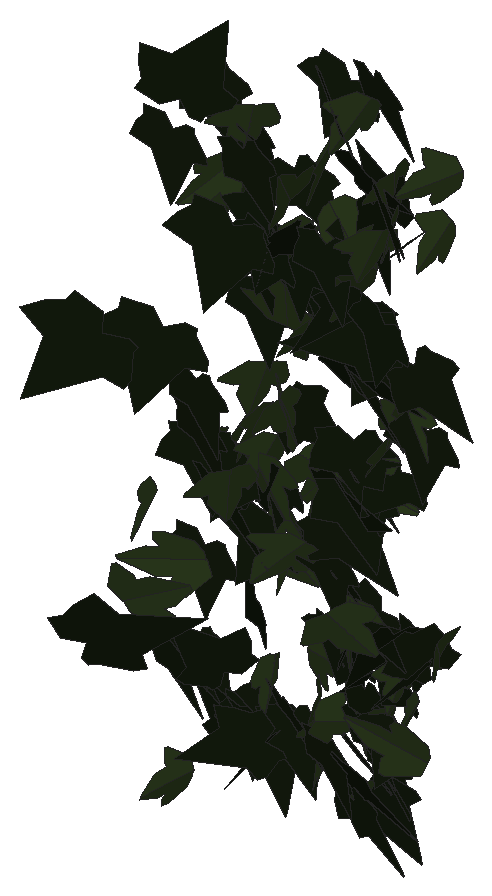
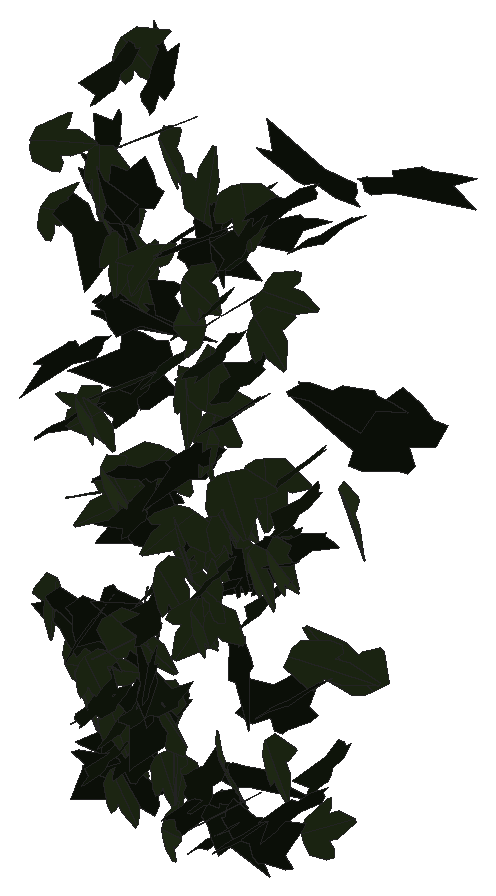
# SketchUp Ruby script. Lengths in inches.
U = 1.inch
M = Sketchup.active_model
def pt(a) = Geom::Point3d.new(a.map { |v| v * U })
def face(e, loops, mat)
  f = e.add_face(loops[0].map { |a| pt(a) })
  loops[1..].each { |l| e.add_face(l.map { |a| pt(a) }).erase! }
  f.material = f.back_material = mat if mat
  f
end
# faces: each face lists its corners as indices into pts; further lists are holes
def faces(e, pts, list, mat = nil) = list.each { |f| face(e, (f[0].is_a?(Array) ? f : [f]).map { |l| l.map { |i| pts[i] } }, mat) }
# xy, xz, yz: faces in a plane at the given z, y or x. An outline is a flat list of corners, or four numbers for a rectangle; further outlines are holes
def ring(l) = l.size == 4 ? [[l[0], l[1]], [l[2], l[1]], [l[2], l[3]], [l[0], l[3]]] : l.each_slice(2).to_a
def flat(e, list, mat, &to3) = list.each { |f| face(e, (f[0].is_a?(Array) ? f : [f]).map { |l| ring(l).map { |u, v| to3.(u, v) } }, mat) }
def xy(e, z, list, mat = nil) = flat(e, list, mat) { |x, y| [x, y, z] }
def xz(e, y, list, mat = nil) = flat(e, list, mat) { |x, z| [x, y, z] }
def yz(e, x, list, mat = nil) = flat(e, list, mat) { |y, z| [x, y, z] }
def lines(e, pts, list) = list.each { |a, b| e.add_line(pt(pts[a]), pt(pts[b])) }
# prism: a flat outline (further loops are holes) pulled along v
def prism(e, loops, v, mat = nil)
  f = face(e, loops, mat); d = Geom::Vector3d.new(v.map { |x| x * U })
  f.pushpull(f.normal.samedirection?(d) ? d.length : -d.length)
end
def box(e, o, s, mat = nil) = prism(e, [[o, [o[0] + s[0], o[1], o[2]], [o[0] + s[0], o[1] + s[1], o[2]], [o[0], o[1] + s[1], o[2]]]], [0, 0, s[2]], mat)
def at(x, y, z, deg = 0) = Geom::Transformation.translation(pt([x, y, z])) * Geom::Transformation.rotation(ORIGIN, Z_AXIS, deg.degrees)
def axes(o, x, y, z) = Geom::Transformation.new([*x, 0, *y, 0, *z, 0, *pt(o).to_a, 1])
def part(name) = M.definitions.add(name)
# library, detail: a bought-in or finely detailed component or shape, given as its bounding box
def library(name, o, s) = part(name).tap { |d| box(d.entities, o, s) }
def detail(e, o, s) = box(e.add_group.entities, o, s)
def put(e, d, t, mat = nil) = e.add_instance(d, t).tap { |i| i.material = mat if mat }
def group(e, t, mat = nil) = e.add_group.tap { |g| g.transformation = t; g.material = mat if mat }.entities
root = M.entities
M.materials.add("1026 AP 7946 SUNNY SIDE UP").color = [254, 231, 186]
M.materials.add("efeu1").color = [18, 25, 13]
M.materials.add("efeu2").color = [43, 57, 29]
c1 = part("ivyleaf_9")
p = [[1.54,2.16,1.25],[1.36,2.04,1.19],[-0.21,0.99,0.68],[-0.71,1.11,0.82],[-0.85,0.86,0.67],[-0.8,0.17,0.21],
  [-0.9,-0.01,0.1],[-0.67,-0.16,-0.02],[-0.08,-0.08,-0.05],[-0.03,-0.6,-0.4],[0.65,-0.88,-0.66],[0.83,-0.6,-0.49],
  [1.29,-0.42,-0.43],[1.8125,-0.07,-0.26],[1.21,0.44,0.15]]
faces(c1.entities,p,[[0,1,2,3,4,5,6,7,8,9,10,11,12,13,14]],"efeu1")
c2 = part("ivyleaf_10")
p = [[0,0.5,-0.03],[-0.0625,2.02,-0.43],[-0.19,2.01,-0.46],[-0.54,1.05,-0.29],[-0.52,0.625,-0.18],[-0.83,0.76,-0.28],
  [-1.16,0.64,-0.33],[-1.15,0.33,-0.24],[-0.77,-0.39,0.02],[-0.3,-0.51,0.16],[0.04,-0.48,0.23],[-0.02,2.01,-0.4375],
  [-0.06,2.01,-0.43],[0.04,-0.49,0.23],[0.67,-0.49,0.14],[1.38,0.36,-0.2],[1.375,0.51,-0.24],[0.81,0.65,-0.19],
  [0.62,0.59,-0.15],[0.6,1.09,-0.28],[0.5,1.23,-0.31]]
faces(c2.entities,p,[[0,1,2,3,4,5,6,7,8,9,10],[11,12,0,13,14,15,16,17,18,19,20]],"efeu2")
put(root,c1,axes([119.27,207.23,283.47],[0.0723,0.01785,0.46303],[0.70235,0.05061,-0.04886],[-0.08206,0.44886,-0.01025]),"1026 AP 7946 SUNNY SIDE UP")
put(root,c1,axes([118.96,207.77,288.06],[-0.55273,-0.26197,0.11681],[-0.11258,-0.09563,-0.45093],[0.43547,-0.35723,0.03168]),"1026 AP 7946 SUNNY SIDE UP")
put(root,c2,axes([121.6,209.79,283.51],[-0.33142,-0.22889,-0.23164],[0.26923,0.14544,-0.31887],[0.42498,-0.27064,0.02137]),"1026 AP 7946 SUNNY SIDE UP")
put(root,c2,axes([118.09,209.97,284.15],[0.24212,-0.34202,-0.03713],[-0.02534,0.03014,-0.38622],[0.53986,0.15481,-0.00147]),"1026 AP 7946 SUNNY SIDE UP")
put(root,c1,axes([119.03,210.66,288.52],[-0.31904,-0.36893,0.03508],[0.00177,-0.04182,-0.43345],[0.58288,-0.2018,0.02052]),"1026 AP 7946 SUNNY SIDE UP")
put(root,c2,axes([117.99,210.81,279.3],[0.00507,-0.02154,0.37214],[0.06882,-0.3587,-0.02453],[0.56503,0.04388,-0.00035]),"1026 AP 7946 SUNNY SIDE UP")
put(root,c1,axes([117.71,210.74,286.4],[-0.47629,-0.266,-0.09673],[0.14411,0.03517,-0.41368],[0.41865,-0.31472,0.03235]),"1026 AP 7946 SUNNY SIDE UP")
put(root,c2,axes([119.04,210.58,284.55],[-0.23896,-0.35345,-0.04487],[0.04278,0.03351,-0.39598],[0.55796,-0.15395,0.01114]),"1026 AP 7946 SUNNY SIDE UP")
put(root,c2,axes([117.3125,210.67,281.95],[-0.39183,-0.04375,0.2858],[0.41038,0.10184,0.25841],[-0.1642,0.35893,-0.03618]),"1026 AP 7946 SUNNY SIDE UP")
put(root,c1,axes([121.41,211.1,287.61],[-0.03806,-0.30393,0.19273],[-0.02274,-0.18825,-0.3152],[0.56214,-0.02819,0.0003]),"1026 AP 7946 SUNNY SIDE UP")
put(root,c1,axes([118.55,211.06,281.09],[0.1272,0.0928,0.35483],[-0.48936,-0.15313,0.1171],[0.27245,-0.31838,0.04466]),"1026 AP 7946 SUNNY SIDE UP")
put(root,c1,axes([119.24,211.25,288.06],[-0.10866,-0.26363,0.23482],[0.00898,-0.2347,-0.27742],[0.54946,-0.0483,0.05097]),"1026 AP 7946 SUNNY SIDE UP")
put(root,c2,axes([120.97,211.16,290.9375],[-0.11826,-0.28478,0.22358],[0.00122,-0.22352,-0.30095],[0.56454,-0.05917,0.04749]),"1026 AP 7946 SUNNY SIDE UP")
put(root,c2,axes([119.76,211.16,283.41],[-0.25485,-0.22405,0.22789],[-0.17352,-0.19411,-0.28534],[0.46518,-0.19516,0.01841]),"1026 AP 7946 SUNNY SIDE UP")
put(root,c1,axes([120.3,211.18,280.42],[0.15225,-0.31296,0.08945],[0.0206,-0.08862,-0.33773],[0.51102,0.09681,-0.01304]),"1026 AP 7946 SUNNY SIDE UP")
put(root,c2,axes([119.6,211.31,288.96],[-0.05659,-0.29494,-0.28113],[-0.03716,-0.27027,0.30443],[-0.62894,0.0425,0.00731]),"1026 AP 7946 SUNNY SIDE UP")
put(root,c1,axes([120.33,211.37,290.57],[-0.01449,-0.11425,0.40246],[0.04558,-0.39061,-0.11907],[0.63937,0.02526,0.01761]),"1026 AP 7946 SUNNY SIDE UP")
put(root,c1,axes([119.11,211.24,280.04],[-0.46237,-0.05005,0.15696],[-0.2235,-0.0673,-0.3052],[0.1177,-0.3244,0.03708]),"1026 AP 7946 SUNNY SIDE UP")
put(root,c1,axes([117.46,211.3125,289.26],[-0.08111,-0.34399,0.06496],[-0.00048,-0.06566,-0.3586],[0.55047,-0.05075,0.00926]),"1026 AP 7946 SUNNY SIDE UP")
put(root,c1,axes([119.65,211.32,288.41],[-0.21655,0.11551,-0.31747],[0.17231,-0.29962,-0.16755],[-0.48898,-0.15674,0.08155]),"1026 AP 7946 SUNNY SIDE UP")
put(root,c1,axes([119.34,211.37,288.67],[-0.21556,0.05674,-0.38318],[0.46434,-0.22964,-0.14943],[-0.36743,-0.32349,0.03596]),"1026 AP 7946 SUNNY SIDE UP")
put(root,c1,axes([117.88,211.32,285.35],[0.08751,-0.33903,0.04372],[0.00471,-0.04446,-0.35417],[0.53761,0.05558,-0.00402]),"1026 AP 7946 SUNNY SIDE UP")
put(root,c1,axes([121.17,211.41,289.31],[0.22112,-0.10123,-0.35227],[0.47956,-0.15517,0.17593],[-0.28894,-0.33501,0.0224]),"1026 AP 7946 SUNNY SIDE UP")
put(root,c1,axes([120.86,211.2,279.66],[0.32279,-0.2569,-0.08403],[-0.07729,0.06327,-0.3384],[0.41601,0.21108,0.00233]),"1026 AP 7946 SUNNY SIDE UP")
put(root,c2,axes([121.82,211.1875,280.81],[-0.14903,-0.01053,-0.36355],[-0.54968,0.05348,0.09541],[0.077,0.36141,-0.02255]),"1026 AP 7946 SUNNY SIDE UP")
put(root,c1,axes([117.84,211.4,284.7],[0.14055,-0.31672,0.10267],[0.03789,-0.09861,-0.33958],[0.52156,0.09251,-0.003]),"1026 AP 7946 SUNNY SIDE UP")
put(root,c1,axes([118.19,211.35,283.84],[0.34368,-0.33159,0.07424],[0.03544,-0.07358,-0.40898],[0.53303,0.21869,-0.02068]),"1026 AP 7946 SUNNY SIDE UP")
put(root,c1,axes([120.58,211.3,280.02],[0.42716,-0.18369,0.14825],[0.16073,-0.10662,-0.33719],[0.33095,0.28886,-0.02758]),"1026 AP 7946 SUNNY SIDE UP")
put(root,c1,axes([118.7,211.38,289.3125],[0.16333,-0.34209,-0.02416],[-0.02073,0.01847,-0.36813],[0.53857,0.10446,-0.00684]),"1026 AP 7946 SUNNY SIDE UP")
put(root,c2,axes([117.68,211.38,282.41],[0.16931,-0.00521,-0.35469],[-0.52703,-0.08413,-0.10717],[-0.12389,0.35077,-0.02881]),"1026 AP 7946 SUNNY SIDE UP")
put(root,c1,axes([120.11,211.46,288.24],[0.02721,-0.35324,0.01497],[0.00014,-0.01655,-0.36444],[0.55605,0.01729,-0.00064]),"1026 AP 7946 SUNNY SIDE UP")
put(root,c1,axes([117.23,211.42,280.86],[0.23734,-0.29354,0.04164],[0.00824,-0.04458,-0.33992],[0.4662,0.15023,-0.01519]),"1026 AP 7946 SUNNY SIDE UP")
put(root,c2,axes([121.04,211.4,288.74],[-0.1834,-0.32732,0.08032],[-0.01571,-0.08108,-0.358],[0.52954,-0.11577,0.0172]),"1026 AP 7946 SUNNY SIDE UP")
put(root,c2,axes([120.1,211.46,289.75],[0.20736,-0.31965,0.13025],[0.06892,-0.12064,-0.35689],[0.53717,0.13887,-0.00449]),"1026 AP 7946 SUNNY SIDE UP")
put(root,c1,axes([117.71,211.2,289.98],[-0.46698,0.1942,0.22772],[0.32132,-0.08767,0.36349],[0.33106,0.35902,-0.03158]),"1026 AP 7946 SUNNY SIDE UP")
put(root,c1,axes([119,211.64,283.17],[-0.28684,-0.25382,0.13022],[-0.02858,-0.14118,-0.31631],[0.44595,-0.1723,0.06348]),"1026 AP 7946 SUNNY SIDE UP")
put(root,c2,axes([119.375,211.32,285.52],[-0.09944,-0.30369,-0.15758],[0.10038,0.14044,-0.31721],[0.52394,-0.08455,0.03087]),"1026 AP 7946 SUNNY SIDE UP")
put(root,c2,axes([120.27,211.2,280.82],[-0.05776,-0.09502,-0.33484],[0.26367,0.2783,-0.10189],[0.46166,-0.17084,0.0163]),"1026 AP 7946 SUNNY SIDE UP")
put(root,c1,axes([117.875,211.54,284.32],[-0.1917,-0.3008,-0.1039],[0.07119,0.0886,-0.33374],[0.49289,-0.12979,0.00779]),"1026 AP 7946 SUNNY SIDE UP")
put(root,c1,axes([120.96,211.61,286.93],[-0.45254,0.00304,0.23472],[-0.35611,-0.04402,-0.29438],[0.03924,-0.36441,0.03535]),"1026 AP 7946 SUNNY SIDE UP")
put(root,c1,axes([120.52,211.68,287.36],[0.021,0.08055,-0.36137],[-0.02984,-0.35083,-0.08568],[-0.56584,0.02149,-0.00889]),"1026 AP 7946 SUNNY SIDE UP")
put(root,c2,axes([120.29,211.72,282.1875],[0.13277,-0.1327,0.33736],[0.34978,-0.24263,-0.16142],[0.43308,0.23664,0.02694]),"1026 AP 7946 SUNNY SIDE UP")
put(root,c2,axes([120.41,211.73,287.49],[-0.11359,-0.24495,-0.26929],[-0.0791,-0.25565,0.26102],[-0.55608,0.0864,0.01788]),"1026 AP 7946 SUNNY SIDE UP")
put(root,c1,axes([120.58,211.61,280.76],[0.24396,-0.27932,-0.01255],[-0.03559,-0.00048,-0.32852],[0.43808,0.15551,-0.0197]),"1026 AP 7946 SUNNY SIDE UP")
put(root,c1,axes([121.1,211.79,280.6],[-0.1552,-0.27336,0.16236],[-0.0242,-0.16238,-0.2981],[0.49679,-0.09331,0.0362]),"1026 AP 7946 SUNNY SIDE UP")
put(root,c2,axes([119.55,211.32,285.18],[-0.15586,0.16681,-0.32485],[-0.2027,0.28947,0.20059],[0.52444,0.16146,-0.01902]),"1026 AP 7946 SUNNY SIDE UP")
put(root,c1,axes([119.86,211.77,283.11],[0.06685,-0.35386,0.0836],[-0.00272,-0.08392,-0.36747],[0.57156,0.04099,-0.01153]),"1026 AP 7946 SUNNY SIDE UP")
put(root,c1,axes([120.2,211.59,283.77],[-0.05483,-0.19776,-0.28665],[0.32329,0.20981,-0.17967],[0.42668,-0.18438,0.0993]),"1026 AP 7946 SUNNY SIDE UP")
put(root,c1,axes([118.85,211.43,282.16],[0.17233,-0.02558,-0.34789],[-0.50876,0.0964,-0.11519],[0.15649,0.34156,0.00863]),"1026 AP 7946 SUNNY SIDE UP")
put(root,c1,axes([121.09,211.7,282.22],[-0.0476,0.24807,-0.26669],[0.05207,-0.25817,-0.25896],[-0.56297,-0.04485,-0.00141]),"1026 AP 7946 SUNNY SIDE UP")
put(root,c2,axes([118.04,211.7,280.93],[0.07461,-0.34398,0.01441],[-0.00343,-0.01639,-0.35779],[0.54145,0.0473,-0.00425]),"1026 AP 7946 SUNNY SIDE UP")
put(root,c1,axes([120.34,211.77,284.22],[-0.08114,-0.32891,-0.12629],[0.06613,0.11533,-0.34155],[0.54694,-0.06274,0.02256]),"1026 AP 7946 SUNNY SIDE UP")
put(root,c1,axes([118.6,211.97,287.92],[-0.18784,-0.24877,0.22669],[-0.07059,-0.2211,-0.2821],[0.51892,-0.12013,0.04368]),"1026 AP 7946 SUNNY SIDE UP")
put(root,c1,axes([120.71,211.7,279.68],[-0.17972,-0.11894,-0.3288],[0.41389,0.1817,-0.16615],[0.33833,-0.28546,0.0286]),"1026 AP 7946 SUNNY SIDE UP")
put(root,c1,axes([121.62,211.77,281.92],[-0.31121,0.18615,-0.17988],[0.12604,-0.16581,-0.27502],[-0.38221,-0.20625,0.05577]),"1026 AP 7946 SUNNY SIDE UP")
put(root,c1,axes([120.55,211.84,279.875],[0.34606,-0.25477,0.02838],[0.00079,0.03864,0.34606],[-0.40318,-0.2186,0.02504]),"1026 AP 7946 SUNNY SIDE UP")
put(root,c1,axes([119.93,211.86,283.92],[0.12855,-0.08863,0.35421],[0.29583,-0.28901,-0.12435],[0.47439,0.20425,-0.01844]),"1026 AP 7946 SUNNY SIDE UP")
put(root,c1,axes([119.14,211.93,287.6],[0.01507,-0.32432,0.14133],[0.02085,-0.13865,-0.33495],[0.55444,0.01403,0.00875]),"1026 AP 7946 SUNNY SIDE UP")
put(root,c2,axes([119.29,211.91,288.04],[0.02238,-0.26559,0.24009],[0.06124,-0.23216,-0.2746],[0.55379,0.03641,0.02066]),"1026 AP 7946 SUNNY SIDE UP")
put(root,c2,axes([118.72,211.73,284.14],[-0.4702,0.12526,-0.14769],[0.18001,-0.09661,-0.33188],[-0.24023,-0.31756,0.04039]),"1026 AP 7946 SUNNY SIDE UP")
put(root,c1,axes([120.09,211.72,286.3125],[0.47502,-0.08576,0.18557],[0.25315,-0.08971,-0.32183],[0.18642,0.34035,-0.03581]),"1026 AP 7946 SUNNY SIDE UP")
put(root,c1,axes([120.66,211.87,290.9375],[0.2439,-0.3204,0.07242],[0.0184,-0.07432,-0.36649],[0.51607,0.15408,-0.02116]),"1026 AP 7946 SUNNY SIDE UP")
put(root,c2,axes([117.82,211.89,284.19],[0.14594,-0.27935,0.17523],[0.06611,-0.16681,-0.30401],[0.51131,0.1013,-0.01071]),"1026 AP 7946 SUNNY SIDE UP")
put(root,c2,axes([118.76,211.87,284.43],[-0.10013,-0.29984,0.15174],[0.01551,-0.15328,-0.31433],[0.52624,-0.05253,0.03813]),"1026 AP 7946 SUNNY SIDE UP")
put(root,c2,axes([120.7,211.81,279.6],[-0.02735,-0.32044,0.0741],[-0.00533,-0.07367,-0.33103],[0.517,-0.01771,0.00051]),"1026 AP 7946 SUNNY SIDE UP")
put(root,c1,axes([118.86,211.81,279.77],[-0.24732,0.23176,-0.21318],[0.15019,-0.18618,-0.28887],[-0.46633,-0.18288,0.02002]),"1026 AP 7946 SUNNY SIDE UP")
put(root,c1,axes([118.25,212,283.82],[-0.25079,-0.26653,0.12546],[-0.06848,-0.11729,-0.31992],[0.45666,-0.16397,0.02093]),"1026 AP 7946 SUNNY SIDE UP")
put(root,c2,axes([118.58,211.92,284.84],[0.10921,-0.32184,0.1678],[0.03749,-0.16327,-0.33999],[0.56725,0.07275,-0.00983]),"1026 AP 7946 SUNNY SIDE UP")
put(root,c2,axes([118.47,211.8,289.6875],[-0.29225,-0.30524,0.02096],[0.00556,-0.02797,-0.36789],[0.48118,-0.18507,0.01698]),"1026 AP 7946 SUNNY SIDE UP")
put(root,c2,axes([117.85,211.96,288.47],[0.13835,0.18126,-0.2982],[-0.27667,-0.23336,-0.20628],[-0.46187,0.19408,0.03424]),"1026 AP 7946 SUNNY SIDE UP")
put(root,c1,axes([117.9,211.96,283.52],[0.12413,-0.32061,0.07462],[0.01418,-0.07422,-0.34047],[0.51728,0.07897,-0.00857]),"1026 AP 7946 SUNNY SIDE UP")
put(root,c1,axes([121.58,211.86,281.89],[-0.0151,0.03674,0.33041],[-0.50678,0.01333,-0.01144],[-0.02281,-0.32039,0.03551]),"1026 AP 7946 SUNNY SIDE UP")
put(root,c2,axes([120.94,211.98,288.93],[0.2507,-0.26976,0.19407],[0.14754,-0.16513,-0.32376],[0.49731,0.18498,-0.00177]),"1026 AP 7946 SUNNY SIDE UP")
put(root,c1,axes([117.71,211.86,289.96],[0.04426,-0.33652,-0.1402],[-0.0208,0.13354,-0.34711],[0.56928,0.03104,-0.00178]),"1026 AP 7946 SUNNY SIDE UP")
put(root,c2,axes([120.75,211.88,280.76],[-0.04993,-0.3275,0.04475],[0.00175,-0.04561,-0.33919],[0.51986,-0.0313,0.00544]),"1026 AP 7946 SUNNY SIDE UP")
put(root,c1,axes([118.73,211.97,279.54],[0.00266,-0.32496,0.0031],[0.00319,-0.00485,-0.3348],[0.51102,0.00172,0.00208]),"1026 AP 7946 SUNNY SIDE UP")
put(root,c1,axes([118.4,212,283.7],[-0.00986,0.07829,0.34962],[0.08456,-0.33469,0.07871],[0.54039,0.0538,-0.00594]),"1026 AP 7946 SUNNY SIDE UP")
put(root,c2,axes([119.07,212.04,282.85],[0.10587,-0.27765,0.21302],[0.12699,-0.19388,-0.29419],[0.53085,0.10175,0.02789]),"1026 AP 7946 SUNNY SIDE UP")
put(root,c1,axes([118.91,212.01,280.25],[0.23623,-0.26016,0.14387],[0.07262,-0.13573,-0.3092],[0.45969,0.15514,-0.02509]),"1026 AP 7946 SUNNY SIDE UP")
put(root,c2,axes([120.56,211.9,282.15],[-0.31543,-0.02273,0.29731],[-0.42343,-0.11464,-0.20271],[0.16763,-0.33236,0.04741]),"1026 AP 7946 SUNNY SIDE UP")
put(root,c1,axes([120.51,212.02,288.74],[-0.18522,-0.01736,-0.37564],[0.56556,-0.07036,-0.11669],[-0.09713,-0.37657,0.03684]),"1026 AP 7946 SUNNY SIDE UP")
put(root,c2,axes([118.61,212.05,280.71],[0.32978,-0.20176,0.23159],[0.22347,-0.17716,-0.2999],[0.42063,0.2523,-0.02224]),"1026 AP 7946 SUNNY SIDE UP")
put(root,c1,axes([120.26,211.99,285.96],[0.29068,-0.27561,0.09882],[0.05006,-0.09568,-0.34141],[0.45695,0.18581,-0.02546]),"1026 AP 7946 SUNNY SIDE UP")
put(root,c2,axes([121.27,211.91,281.02],[0.17149,-0.30029,-0.01772],[-0.02628,0.0104,-0.32883],[0.47207,0.10967,-0.01187]),"1026 AP 7946 SUNNY SIDE UP")
put(root,c1,axes([117.41,212.1,282.2],[-0.06396,-0.33941,0.07238],[0.00933,-0.07335,-0.35228],[0.54555,-0.03854,0.01451]),"1026 AP 7946 SUNNY SIDE UP")
put(root,c1,axes([121.2,212.15,281.72],[-0.13026,-0.0184,0.33457],[-0.19343,-0.30858,-0.05212],[0.47367,-0.13107,0.07073]),"1026 AP 7946 SUNNY SIDE UP")
put(root,c1,axes([120.16,212.01,284.87],[-0.09902,-0.33279,-0.13222],[0.06808,0.1203,-0.34768],[0.55563,-0.07405,0.01904]),"1026 AP 7946 SUNNY SIDE UP")
put(root,c1,axes([119.3,211.76,285.29],[0.14838,-0.15241,-0.32027],[-0.15223,0.29683,-0.17895],[0.52142,0.13003,0.03889]),"1026 AP 7946 SUNNY SIDE UP")
put(root,c1,axes([120.67,212.08,280.05],[0.13697,-0.29361,0.07294],[0.017,-0.07234,-0.31577],[0.47523,0.08722,-0.00972]),"1026 AP 7946 SUNNY SIDE UP")
put(root,c1,axes([120.15,212.09,289.13],[0.14021,-0.15597,0.31466],[0.28939,-0.24562,-0.18546],[0.45651,0.2036,0.02093]),"1026 AP 7946 SUNNY SIDE UP")
put(root,c2,axes([119.71,211.99,280.27],[-0.04954,-0.32992,0.03169],[-0.0002,-0.03277,-0.34161],[0.5213,-0.03137,0.00288]),"1026 AP 7946 SUNNY SIDE UP")
put(root,c2,axes([118.72,212.09,283.34],[0.05302,-0.04502,0.35465],[0.49038,-0.14864,-0.05233],[0.2408,0.31262,0.02848]),"1026 AP 7946 SUNNY SIDE UP")
put(root,c2,axes([120.94,211.89,289.48],[-0.06329,-0.34089,-0.11163],[0.03669,0.10436,-0.35285],[0.56033,-0.04534,0.01049]),"1026 AP 7946 SUNNY SIDE UP")
put(root,c2,axes([121.68,212.2,289.64],[-0.06573,-0.06435,0.35592],[-0.06956,-0.34456,-0.07357],[0.54877,-0.05138,0.03331]),"1026 AP 7946 SUNNY SIDE UP")
put(root,c1,axes([119.14,212,288.89],[0.12691,-0.32789,-0.1228],[0.07912,0.13016,-0.3383],[0.54185,0.05779,0.07816]),"1026 AP 7946 SUNNY SIDE UP")
put(root,c1,axes([120.3,212.11,280.86],[0.18229,-0.33524,0.06396],[0.01363,-0.06466,-0.36557],[0.53647,0.11555,-0.01245]),"1026 AP 7946 SUNNY SIDE UP")
put(root,c1,axes([118.2,212.15,279.78],[-0.04213,-0.31306,0.06447],[-0.00357,-0.06439,-0.32405],[0.50253,-0.0267,0.0031]),"1026 AP 7946 SUNNY SIDE UP")
put(root,c2,axes([119.0625,211.87,282.87],[-0.33738,-0.24502,-0.18694],[0.22939,0.11042,-0.33322],[0.41951,-0.25743,0.03186]),"1026 AP 7946 SUNNY SIDE UP")
put(root,c1,axes([118.25,211.91,279.54],[0.11536,-0.0285,0.33017],[-0.37695,0.21465,0.07742],[-0.33783,-0.24925,0.02636]),"1026 AP 7946 SUNNY SIDE UP")
put(root,c2,axes([120.96,212.1,281.47],[-0.08012,-0.28278,0.14467],[0.07883,-0.14926,-0.28849],[0.4913,-0.02216,0.06988]),"1026 AP 7946 SUNNY SIDE UP")
put(root,c2,axes([121.89,211.79,282.24],[-0.00106,0.24629,0.21947],[-0.24146,0.18623,-0.22268],[-0.4499,-0.10054,0.119]),"1026 AP 7946 SUNNY SIDE UP")
put(root,c1,axes([118.98,212.06,279.99],[-0.00916,-0.33195,-0.12299],[-0.0053,0.11756,-0.3413],[0.55367,-0.00437,-0.0053]),"1026 AP 7946 SUNNY SIDE UP")
put(root,c1,axes([120.09,211.73,280.9],[0.13095,0.30033,0.17866],[0.09167,0.16191,-0.31992],[-0.5362,0.10103,-0.01107]),"1026 AP 7946 SUNNY SIDE UP")
put(root,c1,axes([118.59,212.25,280],[-0.14595,-0.27879,0.15354],[-0.01309,-0.15476,-0.30127],[0.49808,-0.08576,0.03707]),"1026 AP 7946 SUNNY SIDE UP")
put(root,c1,axes([121.3,212.21,285.34],[-0.08471,-0.33035,0.06673],[-0.00885,-0.0666,-0.34517],[0.52984,-0.05393,0.0049]),"1026 AP 7946 SUNNY SIDE UP")
put(root,c1,axes([119.74,212.13,282.7],[0.2771,-0.26575,0.09924],[0.05841,-0.09255,-0.32844],[0.44144,0.17906,-0.01884]),"1026 AP 7946 SUNNY SIDE UP")
put(root,c1,axes([118.65,212.26,283.74],[-0.01119,-0.27159,0.2013],[-0.01404,-0.19676,-0.28102],[0.52732,-0.011,-0.00321]),"1026 AP 7946 SUNNY SIDE UP")
put(root,c2,axes([119.61,211.94,284.15],[0.19632,-0.27843,-0.18781],[-0.15185,0.15427,-0.31267],[0.49938,0.15637,-0.02124]),"1026 AP 7946 SUNNY SIDE UP")
put(root,c2,axes([119.56,212.17,283.4],[0.01197,-0.33755,0.15753],[0.04792,-0.15377,-0.34781],[0.58197,0.0196,0.0254]),"1026 AP 7946 SUNNY SIDE UP")
put(root,c2,axes([118.9,212.04,286.46],[-0.55906,0.02825,0.01301],[0.02176,0.01698,0.36706],[0.0434,0.35536,-0.01647]),"1026 AP 7946 SUNNY SIDE UP")
put(root,c1,axes([118.12,212.2,289.31],[0.22193,-0.30761,0.09988],[0.03289,-0.09878,-0.34855],[0.50691,0.14109,-0.02111]),"1026 AP 7946 SUNNY SIDE UP")
put(root,c1,axes([120.39,212.32,286.1875],[-0.22282,-0.25629,0.1834],[-0.00352,-0.19619,-0.29159],[0.49198,-0.11748,0.08098]),"1026 AP 7946 SUNNY SIDE UP")
put(root,c2,axes([121.52,212.3,288.65],[-0.08882,-0.16662,0.31296],[0.13281,-0.30606,-0.15806],[0.52971,0.0488,0.0921]),"1026 AP 7946 SUNNY SIDE UP")
put(root,c1,axes([119.8,212.33,290.4375],[-0.21126,-0.29214,0.15839],[0.01076,-0.17014,-0.32441],[0.52021,-0.11512,0.07103]),"1026 AP 7946 SUNNY SIDE UP")
put(root,c1,axes([118.33,212.25,286.49],[-0.0237,-0.34009,0.05497],[0.00403,-0.05546,-0.35099],[0.54177,-0.01447,0.00501]),"1026 AP 7946 SUNNY SIDE UP")
put(root,c1,axes([120.35,212.34,282.09],[-0.23557,-0.19978,0.2267],[-0.07975,-0.22687,-0.24781],[0.46184,-0.14108,0.07285]),"1026 AP 7946 SUNNY SIDE UP")
put(root,c2,axes([119.29,212.01,286.45],[-0.03195,-0.35361,-0.13203],[0.02132,0.12556,-0.3641],[0.58995,-0.02369,0.00601]),"1026 AP 7946 SUNNY SIDE UP")
put(root,c1,axes([120.7,212.34,284.44],[-0.31639,-0.22862,0.13195],[0.01567,-0.1695,-0.29358],[0.41276,-0.16881,0.11229]),"1026 AP 7946 SUNNY SIDE UP")
put(root,c1,axes([117.28,212.11,280.59],[0.08398,-0.30541,-0.15444],[-0.03881,0.14612,-0.31855],[0.53235,0.05883,0.00114]),"1026 AP 7946 SUNNY SIDE UP")
put(root,c1,axes([118.14,212.3125,287.05],[0.04985,-0.28433,0.19482],[0.08865,-0.18459,-0.29422],[0.53099,0.05751,0.03084]),"1026 AP 7946 SUNNY SIDE UP")
put(root,c2,axes([119.5,212.01,280.57],[0.14587,-0.28883,-0.14497],[0.01661,0.14746,-0.30736],[0.50379,0.07877,0.05211]),"1026 AP 7946 SUNNY SIDE UP")
put(root,c2,axes([120.86,212.19,285.57],[-0.40928,0.03724,-0.21252],[0.24922,-0.18073,-0.24044],[-0.21622,-0.2788,0.12514]),"1026 AP 7946 SUNNY SIDE UP")
put(root,c1,axes([119.88,212.11,281.27],[-0.01553,0.26919,0.21028],[-0.12936,-0.19847,0.26638],[0.51372,-0.04184,0.07343]),"1026 AP 7946 SUNNY SIDE UP")
put(root,c2,axes([117.8,212.23,288.04],[-0.04388,-0.32182,0.13977],[0.01184,-0.13846,-0.33308],[0.55016,-0.02269,0.01832]),"1026 AP 7946 SUNNY SIDE UP")
put(root,c2,axes([120.46,212.07,288.37],[-0.11148,-0.3353,-0.07935],[0.07281,0.06668,-0.35125],[0.53537,-0.07889,0.03125]),"1026 AP 7946 SUNNY SIDE UP")
put(root,c1,axes([120.92,211.93,288.85],[0.00679,0.00684,0.37477],[-0.21535,0.33704,-0.00288],[-0.52997,-0.13686,0.00597]),"1026 AP 7946 SUNNY SIDE UP")
put(root,c1,axes([119.66,212.4,281.33],[-0.1412,-0.25439,0.25303],[0.10189,-0.26233,-0.25555],[0.54821,-0.01677,0.11267]),"1026 AP 7946 SUNNY SIDE UP")
put(root,c1,axes([121.1,211.85,288.38],[0.06364,0.33308,0.16868],[0.02776,0.16089,-0.34471],[-0.58163,0.04412,0.002]),"1026 AP 7946 SUNNY SIDE UP")
put(root,c2,axes([120.93,212.27,285.69],[0.14441,-0.29133,0.16084],[0.05915,-0.1535,-0.31544],[0.51758,0.09882,-0.00883]),"1026 AP 7946 SUNNY SIDE UP")
put(root,c1,axes([119.35,212.34,286.92],[0.0163,-0.32245,0.13172],[0.02045,-0.1293,-0.33301],[0.54611,0.01447,0.00854]),"1026 AP 7946 SUNNY SIDE UP")
put(root,c1,axes([121.25,212.06,286.44],[0.14194,-0.28099,-0.25365],[-0.05255,0.24457,-0.30069],[0.58344,0.09039,0.03462]),"1026 AP 7946 SUNNY SIDE UP")
put(root,c2,axes([119.86,212.02,288.43],[0.1133,0.34035,0.10906],[0.04484,0.10017,-0.35774],[-0.55776,0.07719,-0.0066]),"1026 AP 7946 SUNNY SIDE UP")
put(root,c2,axes([119.27,212.31,281.06],[0.06356,-0.08892,-0.32998],[0.30279,-0.25613,0.09694],[-0.42513,-0.19572,0.01971]),"1026 AP 7946 SUNNY SIDE UP")
put(root,c2,axes([120.47,212.29,284.76],[0.13876,-0.28371,0.15183],[0.04515,-0.14692,-0.30658],[0.50186,0.09166,-0.0144]),"1026 AP 7946 SUNNY SIDE UP")
put(root,c1,axes([119.96,212.22,284.43],[0.32469,-0.25624,0.02363],[-0.00052,-0.03154,-0.33858],[0.40474,0.20552,-0.01939]),"1026 AP 7946 SUNNY SIDE UP")
put(root,c2,axes([119.34,212.03,284.33],[-0.23574,-0.19732,-0.24125],[0.2938,0.14609,-0.25039],[0.3798,-0.23549,0.04395]),"1026 AP 7946 SUNNY SIDE UP")
put(root,c2,axes([117.92,212.22,284.21],[0.12539,-0.31474,0.04853],[-0.00339,-0.05093,-0.33445],[0.50082,0.07845,-0.01441]),"1026 AP 7946 SUNNY SIDE UP")
put(root,c1,axes([119.8125,212.36,281.57],[-0.09115,0.00483,0.33593],[-0.07656,-0.32758,-0.00583],[0.507,-0.0486,0.05951]),"1026 AP 7946 SUNNY SIDE UP")
put(root,c1,axes([118.52,212.21,287.37],[0.26649,-0.30117,-0.04713],[-0.01606,0.04475,-0.35551],[0.47833,0.16929,0.01432]),"1026 AP 7946 SUNNY SIDE UP")
put(root,c2,axes([119.37,212.36,279.51],[0.09135,-0.16667,0.26484],[0.19225,-0.22835,-0.18165],[0.44309,0.13344,0.02422]),"1026 AP 7946 SUNNY SIDE UP")
put(root,c2,axes([119.22,211.93,287.45],[0.16174,-0.15536,0.32129],[-0.17886,0.29335,0.19038],[-0.51916,-0.14947,0.03451]),"1026 AP 7946 SUNNY SIDE UP")
put(root,c2,axes([118.35,212.23,285.31],[-0.23249,-0.33323,0.05859],[-0.00762,-0.06203,-0.37534],[0.532,-0.14652,0.02023]),"1026 AP 7946 SUNNY SIDE UP")
put(root,c2,axes([120.34,211.94,284.33],[0.11376,0.20647,0.32058],[0.20474,0.28186,-0.22304],[-0.54872,0.14797,-0.01676]),"1026 AP 7946 SUNNY SIDE UP")
put(root,c1,axes([120.58,212.44,281.02],[-0.15154,-0.16786,0.2745],[0.03291,-0.28237,-0.17648],[0.49536,-0.03259,0.0957]),"1026 AP 7946 SUNNY SIDE UP")
